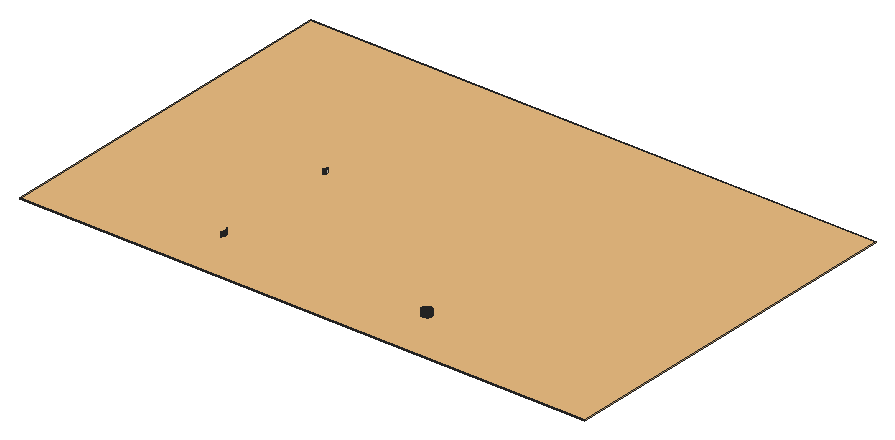
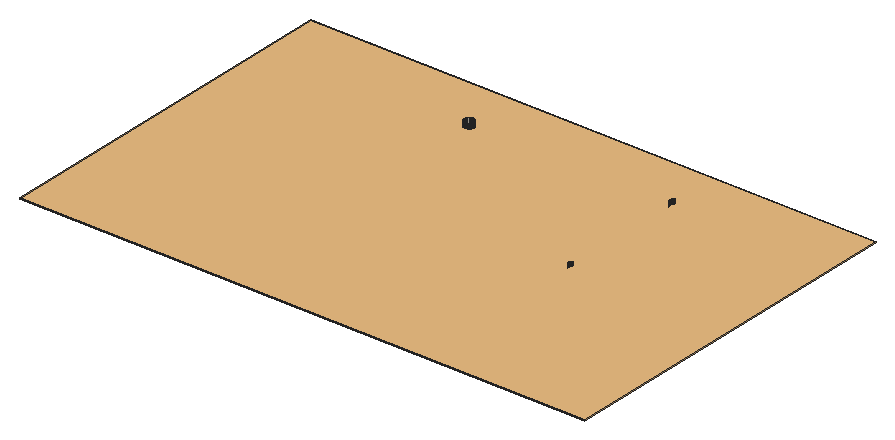
# SketchUp Ruby script. Lengths in inches.
U = 1.inch
M = Sketchup.active_model
def pt(a) = Geom::Point3d.new(a.map { |v| v * U })
def face(e, loops, mat)
  f = e.add_face(loops[0].map { |a| pt(a) })
  loops[1..].each { |l| e.add_face(l.map { |a| pt(a) }).erase! }
  f.material = f.back_material = mat if mat
  f
end
# faces: each face lists its corners as indices into pts; further lists are holes
def faces(e, pts, list, mat = nil) = list.each { |f| face(e, (f[0].is_a?(Array) ? f : [f]).map { |l| l.map { |i| pts[i] } }, mat) }
# xy, xz, yz: faces in a plane at the given z, y or x. An outline is a flat list of corners, or four numbers for a rectangle; further outlines are holes
def ring(l) = l.size == 4 ? [[l[0], l[1]], [l[2], l[1]], [l[2], l[3]], [l[0], l[3]]] : l.each_slice(2).to_a
def flat(e, list, mat, &to3) = list.each { |f| face(e, (f[0].is_a?(Array) ? f : [f]).map { |l| ring(l).map { |u, v| to3.(u, v) } }, mat) }
def xy(e, z, list, mat = nil) = flat(e, list, mat) { |x, y| [x, y, z] }
def xz(e, y, list, mat = nil) = flat(e, list, mat) { |x, z| [x, y, z] }
def yz(e, x, list, mat = nil) = flat(e, list, mat) { |y, z| [x, y, z] }
def lines(e, pts, list) = list.each { |a, b| e.add_line(pt(pts[a]), pt(pts[b])) }
# prism: a flat outline (further loops are holes) pulled along v
def prism(e, loops, v, mat = nil)
  f = face(e, loops, mat); d = Geom::Vector3d.new(v.map { |x| x * U })
  f.pushpull(f.normal.samedirection?(d) ? d.length : -d.length)
end
def box(e, o, s, mat = nil) = prism(e, [[o, [o[0] + s[0], o[1], o[2]], [o[0] + s[0], o[1] + s[1], o[2]], [o[0], o[1] + s[1], o[2]]]], [0, 0, s[2]], mat)
def at(x, y, z, deg = 0) = Geom::Transformation.translation(pt([x, y, z])) * Geom::Transformation.rotation(ORIGIN, Z_AXIS, deg.degrees)
def axes(o, x, y, z) = Geom::Transformation.new([*x, 0, *y, 0, *z, 0, *pt(o).to_a, 1])
def part(name) = M.definitions.add(name)
# library, detail: a bought-in or finely detailed component or shape, given as its bounding box
def library(name, o, s) = part(name).tap { |d| box(d.entities, o, s) }
def detail(e, o, s) = box(e.add_group.entities, o, s)
def put(e, d, t, mat = nil) = e.add_instance(d, t).tap { |i| i.material = mat if mat }
def group(e, t, mat = nil) = e.add_group.tap { |g| g.transformation = t; g.material = mat if mat }.entities
root = M.entities
M.materials.add("0027 AP L140 CRUSHED ICE").color = [241, 233, 217]
M.materials.add("False ceiling Light").color = [253, 207, 127]
c1 = library("Group\#35",[0,0,-0.5],[345,222,0.5])
xz(root,255,[[248.84,120,248.92,123],[248.92,120,249,123],[249,120,249.08,123],[249.08,120,249.16,123]],"0027 AP L140 CRUSHED ICE")
xz(root,261,[[248.84,120,248.92,123],[248.92,120,249,123],[249,120,249.08,123],[249.08,120,249.16,123]],"0027 AP L140 CRUSHED ICE")
yz(root,126,[[257.84,120,257.92,123],[257.92,120,258,123],[258,120,258.08,123],[258.08,120,258.16,123],[335.84,120,335.92,123],
  [335.92,120,336,123]],"0027 AP L140 CRUSHED ICE")
yz(root,246,[[257.84,120,257.92,123],[257.92,120,258,123],[258,120,258.08,123],[258.08,120,258.16,123]],"0027 AP L140 CRUSHED ICE")
yz(root,252,[[257.84,120,257.92,123],[257.92,120,258,123],[258,120,258.08,123],[258.08,120,258.16,123]],"0027 AP L140 CRUSHED ICE")
p = [[248.53,255.04,120],[248.45,255.05,120],[248.45,255.05,123],[248.53,255.04,123],[248.61,255.03,120],[248.61,255.03,123],
  [248.6875,255.02,120],[248.6875,255.02,123],[248.76,255.01,120],[248.76,255.01,123],[248.84,255,120],[248.84,255,123],
  [249.24,255.01,120],[249.16,255,120],[249.16,255,123],[249.24,255.01,123],[249.3125,255.02,120],[249.3125,255.02,123],
  [249.39,255.03,120],[249.39,255.03,123],[249.47,255.04,120],[249.47,255.04,123],[249.55,255.05,120],[249.55,255.05,123],
  [248.07,255.15,120],[248,255.17,120],[248,255.17,123],[248.07,255.15,123],[248.15,255.125,120],[248.15,255.125,123],
  [248.22,255.1,120],[248.22,255.1,123],[248.3,255.08,120],[248.3,255.08,123],[248.375,255.07,120],[248.375,255.07,123],
  [249.625,255.07,120],[249.625,255.07,123],[249.7,255.08,120],[249.7,255.08,123],[249.78,255.1,120],[249.78,255.1,123],
  [249.85,255.125,120],[249.85,255.125,123],[249.93,255.15,120],[249.93,255.15,123],[250,255.17,120],[250,255.17,123],
  [247.85,255.23,120],[247.78,255.26,120],[247.78,255.26,123],[247.85,255.23,123],[247.92,255.2,120],[247.92,255.2,123],
  [250.08,255.2,120],[250.08,255.2,123],[250.15,255.23,120],[250.15,255.23,123],[250.22,255.26,120],[250.22,255.26,123],
  [247.64,255.33,120],[247.57,255.36,120],[247.57,255.36,123],[247.64,255.33,123],[247.71,255.29,120],[247.71,255.29,123],
  [250.29,255.29,120],[250.29,255.29,123],[250.36,255.33,120],[250.36,255.33,123],[250.43,255.36,120],[250.43,255.36,123],
  [247.43,255.44,120],[247.37,255.48,120],[247.37,255.48,123],[247.43,255.44,123],[247.5,255.4,120],[247.5,255.4,123],
  [250.5,255.4,120],[250.5,255.4,123],[250.57,255.44,120],[250.57,255.44,123],[250.63,255.48,120],[250.63,255.48,123],
  [247.3,255.53,120],[247.24,255.57,120],[247.24,255.57,123],[247.3,255.53,123],[250.7,255.53,120],[250.7,255.53,123],
  [250.76,255.57,120],[250.76,255.57,123],[247.17,255.62,120],[247.11,255.67,120],[247.11,255.67,123],[247.17,255.62,123],
  [250.83,255.62,120],[250.83,255.62,123],[250.89,255.67,120],[250.89,255.67,123],[124.95,255.72,120],[124.89,255.67,120],
  [124.89,255.67,123],[124.95,255.72,123],[125.01,255.77,120],[125.01,255.77,123],[247.05,255.72,120],[246.99,255.77,120],
  [246.99,255.77,123],[247.05,255.72,123],[250.95,255.72,120],[250.95,255.72,123],[251.01,255.77,120],[251.01,255.77,123],
  [125.07,255.82,120],[125.07,255.82,123],[125.12,255.88,120],[125.12,255.88,123],[246.93,255.82,120],[246.88,255.88,120],
  [246.88,255.88,123],[246.93,255.82,123],[251.07,255.82,120],[251.07,255.82,123],[251.12,255.88,120],[251.12,255.88,123],
  [125.18,255.93,120],[125.18,255.93,123],[125.23,255.99,120],[125.23,255.99,123],[246.82,255.93,120],[246.77,255.99,120],
  [246.77,255.99,123],[246.82,255.93,123],[251.18,255.93,120],[251.18,255.93,123],[251.23,255.99,120],[251.23,255.99,123],
  [125.28,256.05,120],[125.28,256.05,123],[246.72,256.05,120],[246.72,256.05,123],[251.28,256.05,120],[251.28,256.05,123],
  [125.33,256.11,120],[125.33,256.11,123],[125.38,256.17,120],[125.38,256.17,123],[246.67,256.11,120],[246.62,256.17,120],
  [246.62,256.17,123],[246.67,256.11,123],[251.33,256.11,120],[251.33,256.11,123],[251.38,256.17,120],[251.38,256.17,123],
  [125.43,256.24,120],[125.43,256.24,123],[125.47,256.3,120],[125.47,256.3,123],[246.57,256.24,120],[246.53,256.3,120],
  [246.53,256.3,123],[246.57,256.24,123],[251.43,256.24,120],[251.43,256.24,123],[251.47,256.3,120],[251.47,256.3,123],
  [125.52,256.37,120],[125.52,256.37,123],[246.48,256.37,120],[246.48,256.37,123],[251.52,256.37,120],[251.52,256.37,123],
  [125.56,256.43,120],[125.56,256.43,123],[125.6,256.5,120],[125.6,256.5,123],[246.44,256.43,120],[246.4,256.5,120],
  [246.4,256.5,123],[246.44,256.43,123],[251.56,256.43,120],[251.56,256.43,123],[251.6,256.5,120],[251.6,256.5,123],
  [125.64,256.57,120],[125.64,256.57,123],[246.36,256.57,120],[246.36,256.57,123],[251.64,256.57,120],[251.64,256.57,123],
  [125.67,256.64,120],[125.67,256.64,123],[125.71,256.71,120],[125.71,256.71,123],[246.33,256.64,120],[246.29,256.71,120],
  [246.29,256.71,123],[246.33,256.64,123],[251.67,256.64,120],[251.67,256.64,123],[251.71,256.71,120],[251.71,256.71,123],
  [125.74,256.78,120],[125.74,256.78,123],[246.26,256.78,120],[246.26,256.78,123],[251.74,256.78,120],[251.74,256.78,123],
  [125.77,256.85,120],[125.77,256.85,123],[246.23,256.85,120],[246.23,256.85,123],[251.77,256.85,120],[251.77,256.85,123],
  [125.8,256.92,120],[125.8,256.92,123],[125.83,257,120],[125.83,257,123],[246.2,256.92,120],[246.17,257,120],
  [246.17,257,123],[246.2,256.92,123],[251.8,256.92,120],[251.8,256.92,123],[251.83,257,120],[251.83,257,123],
  [125.85,257.07,120],[125.85,257.07,123],[246.15,257.07,120],[246.15,257.07,123],[251.85,257.07,120],[251.85,257.07,123],
  [125.875,257.15,120],[125.875,257.15,123],[125.9,257.22,120],[125.9,257.22,123],[246.125,257.15,120],[246.1,257.22,120],
  [246.1,257.22,123],[246.125,257.15,123],[251.875,257.15,120],[251.875,257.15,123],[251.9,257.22,120],[251.9,257.22,123],
  [125.92,257.3,120],[125.92,257.3,123],[246.08,257.3,120],[246.08,257.3,123],[251.92,257.3,120],[251.92,257.3,123],
  [125.93,257.375,120],[125.93,257.375,123],[246.07,257.375,120],[246.07,257.375,123],[251.93,257.375,120],[251.93,257.375,123],
  [125.95,257.45,120],[125.95,257.45,123],[246.05,257.45,120],[246.05,257.45,123],[251.95,257.45,120],[251.95,257.45,123],
  [125.96,257.53,120],[125.96,257.53,123],[125.97,257.61,120],[125.97,257.61,123],[246.04,257.53,120],[246.03,257.61,120],
  [246.03,257.61,123],[246.04,257.53,123],[251.96,257.53,120],[251.96,257.53,123],[251.97,257.61,120],[251.97,257.61,123],
  [125.98,257.6875,120],[125.98,257.6875,123],[246.02,257.6875,120],[246.02,257.6875,123],[251.98,257.6875,120],[251.98,257.6875,123],
  [125.99,257.76,120],[125.99,257.76,123],[246.01,257.76,120],[246.01,257.76,123],[251.99,257.76,120],[251.99,257.76,123],
  [126,257.84,120],[126,257.84,123],[246,257.84,120],[246,257.84,123],[252,257.84,120],[252,257.84,123],
  [125.98,258.3125,120],[125.99,258.24,120],[125.99,258.24,123],[125.98,258.3125,123],[126,258.16,120],[126,258.16,123],
  [246,258.16,120],[246.01,258.24,120],[246.01,258.24,123],[246,258.16,123],[246.02,258.3125,120],[246.02,258.3125,123],
  [251.98,258.3125,120],[251.99,258.24,120],[251.99,258.24,123],[251.98,258.3125,123],[252,258.16,120],[252,258.16,123],
  [125.97,258.39,120],[125.97,258.39,123],[246.03,258.39,120],[246.03,258.39,123],[251.97,258.39,120],[251.97,258.39,123],
  [125.96,258.47,120],[125.96,258.47,123],[246.04,258.47,120],[246.04,258.47,123],[251.96,258.47,120],[251.96,258.47,123],
  [125.93,258.625,120],[125.95,258.55,120],[125.95,258.55,123],[125.93,258.625,123],[246.05,258.55,120],[246.05,258.55,123],
  [246.07,258.625,120],[246.07,258.625,123],[251.93,258.625,120],[251.95,258.55,120],[251.95,258.55,123],[251.93,258.625,123],
  [125.92,258.7,120],[125.92,258.7,123],[246.08,258.7,120],[246.08,258.7,123],[251.92,258.7,120],[251.92,258.7,123],
  [125.9,258.78,120],[125.9,258.78,123],[246.1,258.78,120],[246.1,258.78,123],[251.9,258.78,120],[251.9,258.78,123],
  [125.875,258.85,120],[125.875,258.85,123],[246.125,258.85,120],[246.125,258.85,123],[251.875,258.85,120],[251.875,258.85,123],
  [125.83,259,120],[125.85,258.93,120],[125.85,258.93,123],[125.83,259,123],[246.15,258.93,120],[246.15,258.93,123],
  [246.17,259,120],[246.17,259,123],[251.83,259,120],[251.85,258.93,120],[251.85,258.93,123],[251.83,259,123],
  [125.8,259.08,120],[125.8,259.08,123],[246.2,259.08,120],[246.2,259.08,123],[251.8,259.08,120],[251.8,259.08,123],
  [125.74,259.22,120],[125.77,259.15,120],[125.77,259.15,123],[125.74,259.22,123],[246.23,259.15,120],[246.23,259.15,123],
  [246.26,259.22,120],[246.26,259.22,123],[251.74,259.22,120],[251.77,259.15,120],[251.77,259.15,123],[251.74,259.22,123],
  [125.71,259.29,120],[125.71,259.29,123],[246.29,259.29,120],[246.29,259.29,123],[251.71,259.29,120],[251.71,259.29,123],
  [125.67,259.36,120],[125.67,259.36,123],[246.33,259.36,120],[246.33,259.36,123],[251.67,259.36,120],[251.67,259.36,123],
  [125.6,259.5,120],[125.64,259.43,120],[125.64,259.43,123],[125.6,259.5,123],[246.36,259.43,120],[246.36,259.43,123],
  [246.4,259.5,120],[246.4,259.5,123],[251.6,259.5,120],[251.64,259.43,120],[251.64,259.43,123],[251.6,259.5,123],
  [125.56,259.57,120],[125.56,259.57,123],[246.44,259.57,120],[246.44,259.57,123],[251.56,259.57,120],[251.56,259.57,123],
  [125.47,259.7,120],[125.52,259.63,120],[125.52,259.63,123],[125.47,259.7,123],[246.48,259.63,120],[246.48,259.63,123],
  [246.53,259.7,120],[246.53,259.7,123],[251.47,259.7,120],[251.52,259.63,120],[251.52,259.63,123],[251.47,259.7,123],
  [125.43,259.76,120],[125.43,259.76,123],[246.57,259.76,120],[246.57,259.76,123],[251.43,259.76,120],[251.43,259.76,123],
  [125.33,259.89,120],[125.38,259.83,120],[125.38,259.83,123],[125.33,259.89,123],[246.62,259.83,120],[246.62,259.83,123],
  [246.67,259.89,120],[246.67,259.89,123],[251.33,259.89,120],[251.38,259.83,120],[251.38,259.83,123],[251.33,259.89,123],
  [125.23,260.01,120],[125.28,259.95,120],[125.28,259.95,123],[125.23,260.01,123],[246.72,259.95,120],[246.72,259.95,123],
  [246.77,260.01,120],[246.77,260.01,123],[251.23,260.01,120],[251.28,259.95,120],[251.28,259.95,123],[251.23,260.01,123],
  [125.18,260.07,120],[125.18,260.07,123],[246.82,260.07,120],[246.82,260.07,123],[251.18,260.07,120],[251.18,260.07,123],
  [125.07,260.18,120],[125.12,260.12,120],[125.12,260.12,123],[125.07,260.18,123],[246.88,260.12,120],[246.88,260.12,123],
  [246.93,260.18,120],[246.93,260.18,123],[251.07,260.18,120],[251.12,260.12,120],[251.12,260.12,123],[251.07,260.18,123],
  [124.95,260.28,120],[125.01,260.23,120],[125.01,260.23,123],[124.95,260.28,123],[246.99,260.23,120],[246.99,260.23,123],
  [247.05,260.28,120],[247.05,260.28,123],[250.95,260.28,120],[251.01,260.23,120],[251.01,260.23,123],[250.95,260.28,123],
  [124.89,260.33,120],[124.89,260.33,123],[247.11,260.33,120],[247.11,260.33,123],[247.17,260.38,120],[247.17,260.38,123],
  [250.83,260.38,120],[250.89,260.33,120],[250.89,260.33,123],[250.83,260.38,123],[247.24,260.43,120],[247.24,260.43,123],
  [247.3,260.47,120],[247.3,260.47,123],[250.7,260.47,120],[250.76,260.43,120],[250.76,260.43,123],[250.7,260.47,123],
  [247.37,260.52,120],[247.37,260.52,123],[247.43,260.56,120],[247.43,260.56,123],[250.57,260.56,120],[250.63,260.52,120],
  [250.63,260.52,123],[250.57,260.56,123],[247.5,260.6,120],[247.5,260.6,123],[247.57,260.64,120],[247.57,260.64,123],
  [247.64,260.67,120],[247.64,260.67,123],[250.36,260.67,120],[250.43,260.64,120],[250.43,260.64,123],[250.36,260.67,123],
  [250.5,260.6,120],[250.5,260.6,123],[247.71,260.71,120],[247.71,260.71,123],[247.78,260.74,120],[247.78,260.74,123],
  [247.85,260.77,120],[247.85,260.77,123],[250.15,260.77,120],[250.22,260.74,120],[250.22,260.74,123],[250.15,260.77,123],
  [250.29,260.71,120],[250.29,260.71,123],[247.92,260.8,120],[247.92,260.8,123],[248,260.83,120],[248,260.83,123],
  [248.07,260.85,120],[248.07,260.85,123],[249.93,260.85,120],[250,260.83,120],[250,260.83,123],[249.93,260.85,123],
  [250.08,260.8,120],[250.08,260.8,123],[248.15,260.875,120],[248.15,260.875,123],[248.22,260.9,120],[248.22,260.9,123],
  [248.3,260.92,120],[248.3,260.92,123],[248.375,260.93,120],[248.375,260.93,123],[248.45,260.95,120],[248.45,260.95,123],
  [248.53,260.96,120],[248.53,260.96,123],[249.47,260.96,120],[249.55,260.95,120],[249.55,260.95,123],[249.47,260.96,123],
  [249.625,260.93,120],[249.625,260.93,123],[249.7,260.92,120],[249.7,260.92,123],[249.78,260.9,120],[249.78,260.9,123],
  [249.85,260.875,120],[249.85,260.875,123],[248.61,260.97,120],[248.61,260.97,123],[248.6875,260.98,120],[248.6875,260.98,123],
  [248.76,260.99,120],[248.76,260.99,123],[248.84,261,120],[248.84,261,123],[249.16,261,120],[249.24,260.99,120],
  [249.24,260.99,123],[249.16,261,123],[249.3125,260.98,120],[249.3125,260.98,123],[249.39,260.97,120],[249.39,260.97,123],
  [124.95,333.72,120],[124.89,333.67,120],[124.89,333.67,123],[124.95,333.72,123],[125.01,333.77,120],[125.01,333.77,123],
  [125.07,333.82,120],[125.07,333.82,123],[125.12,333.88,120],[125.12,333.88,123],[125.18,333.93,120],[125.18,333.93,123],
  [125.23,333.99,120],[125.23,333.99,123],[125.28,334.05,120],[125.28,334.05,123],[125.33,334.11,120],[125.33,334.11,123],
  [125.38,334.17,120],[125.38,334.17,123],[125.43,334.24,120],[125.43,334.24,123],[125.47,334.3,120],[125.47,334.3,123],
  [125.52,334.37,120],[125.52,334.37,123],[125.56,334.43,120],[125.56,334.43,123],[125.6,334.5,120],[125.6,334.5,123],
  [125.64,334.57,120],[125.64,334.57,123],[125.67,334.64,120],[125.67,334.64,123],[125.71,334.71,120],[125.71,334.71,123],
  [125.74,334.78,120],[125.74,334.78,123],[125.77,334.85,120],[125.77,334.85,123],[125.8,334.92,120],[125.8,334.92,123],
  [125.83,335,120],[125.83,335,123],[125.85,335.07,120],[125.85,335.07,123],[125.875,335.15,120],[125.875,335.15,123],
  [125.9,335.22,120],[125.9,335.22,123],[125.92,335.3,120],[125.92,335.3,123],[125.93,335.375,120],[125.93,335.375,123],
  [125.95,335.45,120],[125.95,335.45,123],[125.96,335.53,120],[125.96,335.53,123],[125.97,335.61,120],[125.97,335.61,123],
  [125.98,335.6875,120],[125.98,335.6875,123],[125.99,335.76,120],[125.99,335.76,123],[126,335.84,120],[126,335.84,123]]
faces(root,p,[[0,1,2,3],[4,0,3,5],[6,4,5,7],[8,6,7,9],[10,8,9,11],[12,13,14,15],[16,12,15,17],[18,16,17,19],
  [20,18,19,21],[22,20,21,23],[24,25,26,27],[28,24,27,29],[30,28,29,31],[32,30,31,33],[34,32,33,35],[1,34,35,2],
  [36,22,23,37],[38,36,37,39],[40,38,39,41],[42,40,41,43],[44,42,43,45],[46,44,45,47],[48,49,50,51],[52,48,51,53],
  [25,52,53,26],[54,46,47,55],[56,54,55,57],[58,56,57,59],[60,61,62,63],[64,60,63,65],[49,64,65,50],[66,58,59,67],
  [68,66,67,69],[70,68,69,71],[72,73,74,75],[76,72,75,77],[61,76,77,62],[78,70,71,79],[80,78,79,81],[82,80,81,83],
  [84,85,86,87],[73,84,87,74],[88,82,83,89],[90,88,89,91],[92,93,94,95],[85,92,95,86],[96,90,91,97],[98,96,97,99],
  [100,101,102,103],[104,100,103,105],[106,107,108,109],[93,106,109,94],[110,98,99,111],[112,110,111,113],[114,104,105,115],[116,114,115,117],
  [118,119,120,121],[107,118,121,108],[122,112,113,123],[124,122,123,125],[126,116,117,127],[128,126,127,129],[130,131,132,133],[119,130,133,120],
  [134,124,125,135],[136,134,135,137],[138,128,129,139],[131,140,141,132],[142,136,137,143],[144,138,139,145],[146,144,145,147],[148,149,150,151],
  [140,148,151,141],[152,142,143,153],[154,152,153,155],[156,146,147,157],[158,156,157,159],[160,161,162,163],[149,160,163,150],[164,154,155,165],
  [166,164,165,167],[168,158,159,169],[161,170,171,162],[172,166,167,173],[174,168,169,175],[176,174,175,177],[178,179,180,181],[170,178,181,171],
  [182,172,173,183],[184,182,183,185],[186,176,177,187],[179,188,189,180],[190,184,185,191],[192,186,187,193],[194,192,193,195],[196,197,198,199],
  [188,196,199,189],[200,190,191,201],[202,200,201,203],[204,194,195,205],[197,206,207,198],[208,202,203,209],[210,204,205,211],[206,212,213,207],
  [214,208,209,215],[216,210,211,217],[218,216,217,219],[220,221,222,223],[212,220,223,213],[224,214,215,225],[226,224,225,227],[228,218,219,229],
  [221,230,231,222],[232,226,227,233],[234,228,229,235],[236,234,235,237],[238,239,240,241],[230,238,241,231],[242,232,233,243],[244,242,243,245],
  [246,236,237,247],[239,248,249,240],[250,244,245,251],[252,246,247,253],[248,254,255,249],[256,250,251,257],[258,252,253,259],[254,260,261,255],
  [262,256,257,263],[264,258,259,265],[266,264,265,267],[268,269,270,271],[260,268,271,261],[272,262,263,273],[274,272,273,275],[276,266,267,277],
  [269,278,279,270],[280,274,275,281],[282,276,277,283],[278,284,285,279],[286,280,281,287],[288,282,283,289],[284,290,291,285],[292,286,287,293],
  [294,295,296,297],[295,298,299,296],[300,301,302,303],[301,304,305,302],[306,307,308,309],[307,310,311,308],[312,294,297,313],[304,314,315,305],
  [316,306,309,317],[318,312,313,319],[314,320,321,315],[322,316,317,323],[324,325,326,327],[325,318,319,326],[320,328,329,321],[328,330,331,329],
  [332,333,334,335],[333,322,323,334],[336,324,327,337],[330,338,339,331],[340,332,335,341],[342,336,337,343],[338,344,345,339],[346,340,341,347],
  [348,342,343,349],[344,350,351,345],[352,346,347,353],[354,355,356,357],[355,348,349,356],[350,358,359,351],[358,360,361,359],[362,363,364,365],
  [363,352,353,364],[366,354,357,367],[360,368,369,361],[370,362,365,371],[372,373,374,375],[373,366,367,374],[368,376,377,369],[376,378,379,377],
  [380,381,382,383],[381,370,371,382],[384,372,375,385],[378,386,387,379],[388,380,383,389],[390,384,385,391],[386,392,393,387],[394,388,389,395],
  [396,397,398,399],[397,390,391,398],[392,400,401,393],[400,402,403,401],[404,405,406,407],[405,394,395,406],[408,396,399,409],[402,410,411,403],
  [412,404,407,413],[414,415,416,417],[415,408,409,416],[410,418,419,411],[418,420,421,419],[422,423,424,425],[423,412,413,424],[426,414,417,427],
  [420,428,429,421],[430,422,425,431],[432,433,434,435],[433,426,427,434],[428,436,437,429],[436,438,439,437],[440,441,442,443],[441,430,431,442],
  [444,445,446,447],[445,432,435,446],[438,448,449,439],[448,450,451,449],[452,453,454,455],[453,440,443,454],[456,444,447,457],[450,458,459,451],
  [460,452,455,461],[462,463,464,465],[463,456,457,464],[458,466,467,459],[466,468,469,467],[470,471,472,473],[471,460,461,472],[474,475,476,477],
  [475,462,465,476],[468,478,479,469],[478,480,481,479],[482,483,484,485],[483,470,473,484],[486,474,477,487],[480,488,489,481],[488,490,491,489],
  [492,493,494,495],[493,482,485,494],[490,496,497,491],[496,498,499,497],[500,501,502,503],[501,492,495,502],[498,504,505,499],[504,506,507,505],
  [508,509,510,511],[509,500,503,510],[506,512,513,507],[512,514,515,513],[514,516,517,515],[518,519,520,521],[519,522,523,520],[522,508,511,523],
  [516,524,525,517],[524,526,527,525],[526,528,529,527],[530,531,532,533],[531,534,535,532],[534,518,521,535],[528,536,537,529],[536,538,539,537],
  [538,540,541,539],[542,543,544,545],[543,546,547,544],[546,530,533,547],[540,548,549,541],[548,550,551,549],[550,552,553,551],[552,554,555,553],
  [554,556,557,555],[556,558,559,557],[560,561,562,563],[561,564,565,562],[564,566,567,565],[566,568,569,567],[568,570,571,569],[570,542,545,571],
  [558,572,573,559],[572,574,575,573],[574,576,577,575],[576,578,579,577],[580,581,582,583],[581,584,585,582],[584,586,587,585],[586,560,563,587],
  [588,589,590,591],[592,588,591,593],[594,592,593,595],[596,594,595,597],[598,596,597,599],[600,598,599,601],[602,600,601,603],[604,602,603,605],
  [606,604,605,607],[608,606,607,609],[610,608,609,611],[612,610,611,613],[614,612,613,615],[616,614,615,617],[618,616,617,619],[620,618,619,621],
  [622,620,621,623],[624,622,623,625],[626,624,625,627],[628,626,627,629],[630,628,629,631],[632,630,631,633],[634,632,633,635],[636,634,635,637],
  [638,636,637,639],[640,638,639,641],[642,640,641,643],[644,642,643,645],[646,644,645,647],[648,646,647,649],[650,648,649,651],[652,650,651,653]],"0027 AP L140 CRUSHED ICE")
put(root,c1,at(27,225,120.5),"False ceiling Light")
